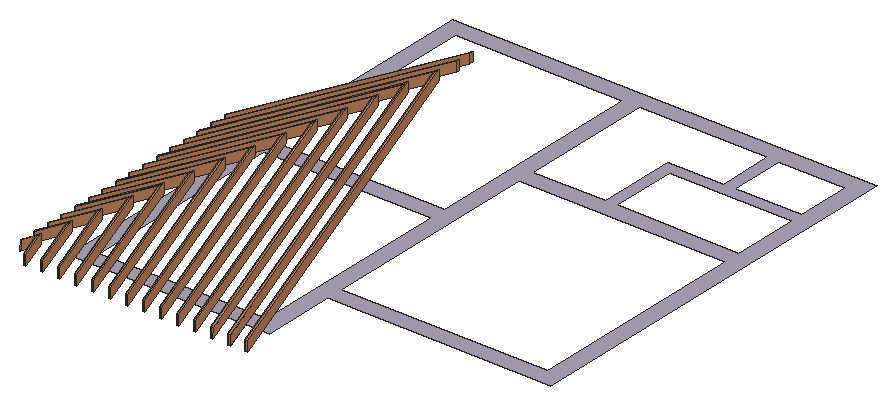
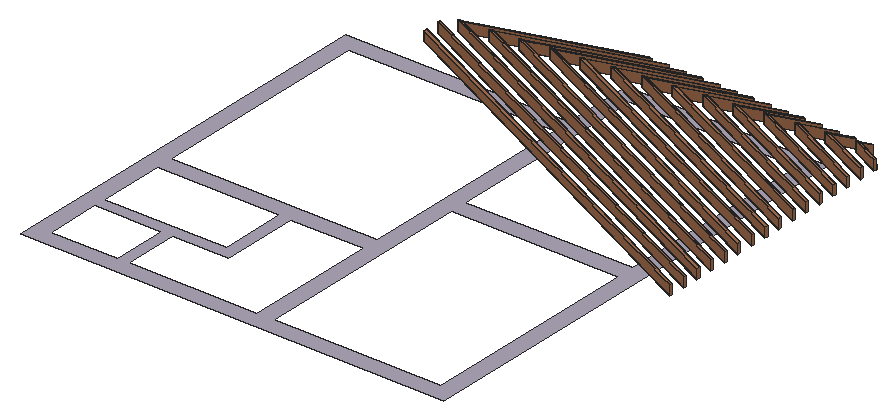
# SketchUp Ruby script. Lengths in millimetres.
U = 1.mm
M = Sketchup.active_model
def pt(a) = Geom::Point3d.new(a.map { |v| v * U })
def face(e, loops, mat)
  f = e.add_face(loops[0].map { |a| pt(a) })
  loops[1..].each { |l| e.add_face(l.map { |a| pt(a) }).erase! }
  f.material = f.back_material = mat if mat
  f
end
# faces: each face lists its corners as indices into pts; further lists are holes
def faces(e, pts, list, mat = nil) = list.each { |f| face(e, (f[0].is_a?(Array) ? f : [f]).map { |l| l.map { |i| pts[i] } }, mat) }
# xy, xz, yz: faces in a plane at the given z, y or x. An outline is a flat list of corners, or four numbers for a rectangle; further outlines are holes
def ring(l) = l.size == 4 ? [[l[0], l[1]], [l[2], l[1]], [l[2], l[3]], [l[0], l[3]]] : l.each_slice(2).to_a
def flat(e, list, mat, &to3) = list.each { |f| face(e, (f[0].is_a?(Array) ? f : [f]).map { |l| ring(l).map { |u, v| to3.(u, v) } }, mat) }
def xy(e, z, list, mat = nil) = flat(e, list, mat) { |x, y| [x, y, z] }
def xz(e, y, list, mat = nil) = flat(e, list, mat) { |x, z| [x, y, z] }
def yz(e, x, list, mat = nil) = flat(e, list, mat) { |y, z| [x, y, z] }
def lines(e, pts, list) = list.each { |a, b| e.add_line(pt(pts[a]), pt(pts[b])) }
# prism: a flat outline (further loops are holes) pulled along v
def prism(e, loops, v, mat = nil)
  f = face(e, loops, mat); d = Geom::Vector3d.new(v.map { |x| x * U })
  f.pushpull(f.normal.samedirection?(d) ? d.length : -d.length)
end
def box(e, o, s, mat = nil) = prism(e, [[o, [o[0] + s[0], o[1], o[2]], [o[0] + s[0], o[1] + s[1], o[2]], [o[0], o[1] + s[1], o[2]]]], [0, 0, s[2]], mat)
def at(x, y, z, deg = 0) = Geom::Transformation.translation(pt([x, y, z])) * Geom::Transformation.rotation(ORIGIN, Z_AXIS, deg.degrees)
def axes(o, x, y, z) = Geom::Transformation.new([*x, 0, *y, 0, *z, 0, *pt(o).to_a, 1])
def part(name) = M.definitions.add(name)
# library, detail: a bought-in or finely detailed component or shape, given as its bounding box
def library(name, o, s) = part(name).tap { |d| box(d.entities, o, s) }
def detail(e, o, s) = box(e.add_group.entities, o, s)
def put(e, d, t, mat = nil) = e.add_instance(d, t).tap { |i| i.material = mat if mat }
def group(e, t, mat = nil) = e.add_group.tap { |g| g.transformation = t; g.material = mat if mat }.entities
root = M.entities
M.materials.add("0268 AP 7144 ITALIAN IRIS").color = [172, 166, 184]
M.materials.add("[Wood Veneer 02]").color = [190, 128, 91]
c1 = part("Group163\#1")
xy(c1.entities,0,[[-381.6,-330.5,-322.7,-279.5,0,-279.5,0,-330.5]])
xy(c1.entities,152,[[-469.4,-330.5,-87.8,-330.5,-87.8,-279.5,-410.5,-279.5]])
xz(c1.entities,-330.5,[[-381.6,0,0,0,-87.8,152,-469.4,152]])
xz(c1.entities,-279.5,[[-322.7,0,-410.5,152,-87.8,152,0,0]])
p = [[-322.7,-279.5,0],[-381.6,-330.5,0],[-469.4,-330.5,152],[-410.5,-279.5,152],[0,-330.5,0],[0,-279.5,0],
  [-87.8,-279.5,152],[-87.8,-330.5,152]]
faces(c1.entities,p,[[0,1,2,3],[4,5,6,7]])
c2 = part("Group214\#1")
xy(c2.entities,0,[[-322.7,-8540.5,-381.6,-8489.5,0,-8489.5,0,-8540.5]])
xy(c2.entities,152,[[-410.5,-8540.5,-87.8,-8540.5,-87.8,-8489.5,-469.4,-8489.5]])
xz(c2.entities,-8540.5,[[-322.7,0,0,0,-87.8,152,-410.5,152]])
xz(c2.entities,-8489.5,[[-381.6,0,-469.4,152,-87.8,152,0,0]])
p = [[-322.7,-8540.5,0],[-410.5,-8540.5,152],[-469.4,-8489.5,152],[-381.6,-8489.5,0],[-87.8,-8540.5,152],[0,-8540.5,0],
  [0,-8489.5,0],[-87.8,-8489.5,152]]
faces(c2.entities,p,[[0,1,2,3],[4,5,6,7]])
c3 = part("Group165\#1")
xy(c3.entities,0,[[-733.8,-635.5,-674.9,-584.5,0,-584.5,0,-635.5]])
xy(c3.entities,152,[[-821.6,-635.5,-87.8,-635.5,-87.8,-584.5,-762.7,-584.5]])
xz(c3.entities,-635.5,[[-733.8,0,0,0,-87.8,152,-821.6,152]])
xz(c3.entities,-584.5,[[-674.9,0,-762.7,152,-87.8,152,0,0]])
p = [[-821.6,-635.5,152],[-762.7,-584.5,152],[-674.9,-584.5,0],[-733.8,-635.5,0],[-87.8,-584.5,152],[-87.8,-635.5,152],
  [0,-635.5,0],[0,-584.5,0]]
faces(c3.entities,p,[[0,1,2,3],[4,5,6,7]])
c4 = part("Group167\#1")
xy(c4.entities,0,[[-1086,-940.5,-1027.1,-889.5,0,-889.5,0,-940.5]])
xy(c4.entities,152,[[-1173.8,-940.5,-87.8,-940.5,-87.8,-889.5,-1114.9,-889.5]])
xz(c4.entities,-940.5,[[-1086,0,0,0,-87.8,152,-1173.8,152]])
xz(c4.entities,-889.5,[[-1027.1,0,-1114.9,152,-87.8,152,0,0]])
p = [[-1114.9,-889.5,152],[-1027.1,-889.5,0],[-1086,-940.5,0],[-1173.8,-940.5,152],[0,-889.5,0],[-87.8,-889.5,152],
  [-87.8,-940.5,152],[0,-940.5,0]]
faces(c4.entities,p,[[0,1,2,3],[4,5,6,7]])
c5 = part("Group216\#1")
xy(c5.entities,0,[[-674.9,-8235.5,-733.8,-8184.5,0,-8184.5,0,-8235.5]])
xy(c5.entities,152,[[-762.7,-8235.5,-87.8,-8235.5,-87.8,-8184.5,-821.6,-8184.5]])
xz(c5.entities,-8235.5,[[-674.9,0,0,0,-87.8,152,-762.7,152]])
xz(c5.entities,-8184.5,[[-733.8,0,-821.6,152,-87.8,152,0,0]])
p = [[-821.6,-8184.5,152],[-733.8,-8184.5,0],[-674.9,-8235.5,0],[-762.7,-8235.5,152],[0,-8184.5,0],[-87.8,-8184.5,152],
  [-87.8,-8235.5,152],[0,-8235.5,0]]
faces(c5.entities,p,[[0,1,2,3],[4,5,6,7]])
c6 = part("Group169\#1")
xy(c6.entities,0,[[-1438.2,-1245.5,-1379.3,-1194.5,0,-1194.5,0,-1245.5]])
xy(c6.entities,152,[[-1525.9,-1245.5,-87.8,-1245.5,-87.8,-1194.5,-1467,-1194.5]])
xz(c6.entities,-1245.5,[[-1438.2,0,0,0,-87.8,152,-1525.9,152]])
xz(c6.entities,-1194.5,[[-1379.3,0,-1467,152,-87.8,152,0,0]])
p = [[-1379.3,-1194.5,0],[-1438.2,-1245.5,0],[-1525.9,-1245.5,152],[-1467,-1194.5,152],[0,-1245.5,0],[0,-1194.5,0],
  [-87.8,-1194.5,152],[-87.8,-1245.5,152]]
faces(c6.entities,p,[[0,1,2,3],[4,5,6,7]])
c7 = part("Group171\#1")
xy(c7.entities,0,[[-1790.4,-1550.5,-1731.5,-1499.5,0,-1499.5,0,-1550.5]])
xy(c7.entities,152,[[-1878.1,-1550.5,-87.8,-1550.5,-87.8,-1499.5,-1819.2,-1499.5]])
xz(c7.entities,-1550.5,[[-1790.4,0,0,0,-87.8,152,-1878.1,152]])
xz(c7.entities,-1499.5,[[-1731.5,0,-1819.2,152,-87.8,152,0,0]])
p = [[-1819.2,-1499.5,152],[-1731.5,-1499.5,0],[-1790.4,-1550.5,0],[-1878.1,-1550.5,152],[0,-1499.5,0],[-87.8,-1499.5,152],
  [-87.8,-1550.5,152],[0,-1550.5,0]]
faces(c7.entities,p,[[0,1,2,3],[4,5,6,7]])
c8 = part("Group218\#1")
xy(c8.entities,0,[[-1027.1,-7930.5,-1086,-7879.5,0,-7879.5,0,-7930.5]])
xy(c8.entities,152,[[-1114.9,-7930.5,-87.8,-7930.5,-87.8,-7879.5,-1173.8,-7879.5]])
xz(c8.entities,-7930.5,[[-1027.1,0,0,0,-87.8,152,-1114.9,152]])
xz(c8.entities,-7879.5,[[-1086,0,-1173.8,152,-87.8,152,0,0]])
p = [[-1173.8,-7879.5,152],[-1086,-7879.5,0],[-1027.1,-7930.5,0],[-1114.9,-7930.5,152],[0,-7879.5,0],[-87.8,-7879.5,152],
  [-87.8,-7930.5,152],[0,-7930.5,0]]
faces(c8.entities,p,[[0,1,2,3],[4,5,6,7]])
c9 = part("Group173\#1")
xy(c9.entities,0,[[-2142.5,-1855.5,-2083.7,-1804.5,0,-1804.5,0,-1855.5]])
xy(c9.entities,152,[[-2230.3,-1855.5,-87.8,-1855.5,-87.8,-1804.5,-2171.4,-1804.5]])
xz(c9.entities,-1855.5,[[-2142.5,0,0,0,-87.8,152,-2230.3,152]])
xz(c9.entities,-1804.5,[[-2083.7,0,-2171.4,152,-87.8,152,0,0]])
p = [[-2083.7,-1804.5,0],[-2142.5,-1855.5,0],[-2230.3,-1855.5,152],[-2171.4,-1804.5,152],[0,-1855.5,0],[0,-1804.5,0],
  [-87.8,-1804.5,152],[-87.8,-1855.5,152]]
faces(c9.entities,p,[[0,1,2,3],[4,5,6,7]])
c10 = part("Group175\#1")
xy(c10.entities,0,[[-2494.7,-2160.5,-2435.8,-2109.5,0,-2109.5,0,-2160.5]])
xy(c10.entities,152,[[-2582.5,-2160.5,-87.8,-2160.5,-87.8,-2109.5,-2523.6,-2109.5]])
xz(c10.entities,-2160.5,[[-2494.7,0,0,0,-87.8,152,-2582.5,152]])
xz(c10.entities,-2109.5,[[-2435.8,0,-2523.6,152,-87.8,152,0,0]])
p = [[-2494.7,-2160.5,0],[-2582.5,-2160.5,152],[-2523.6,-2109.5,152],[-2435.8,-2109.5,0],[-87.8,-2160.5,152],[0,-2160.5,0],
  [0,-2109.5,0],[-87.8,-2109.5,152]]
faces(c10.entities,p,[[0,1,2,3],[4,5,6,7]])
c11 = part("Group220\#1")
xy(c11.entities,0,[[-1379.3,-7625.5,-1438.2,-7574.5,0,-7574.5,0,-7625.5]])
xy(c11.entities,152,[[-1467,-7625.5,-87.8,-7625.5,-87.8,-7574.5,-1525.9,-7574.5]])
xz(c11.entities,-7625.5,[[-1379.3,0,0,0,-87.8,152,-1467,152]])
xz(c11.entities,-7574.5,[[-1438.2,0,-1525.9,152,-87.8,152,0,0]])
p = [[-1379.3,-7625.5,0],[-1467,-7625.5,152],[-1525.9,-7574.5,152],[-1438.2,-7574.5,0],[-87.8,-7625.5,152],[0,-7625.5,0],
  [0,-7574.5,0],[-87.8,-7574.5,152]]
faces(c11.entities,p,[[0,1,2,3],[4,5,6,7]])
c12 = part("Group177\#1")
xy(c12.entities,0,[[-2846.9,-2465.5,-2788,-2414.5,0,-2414.5,0,-2465.5]])
xy(c12.entities,152,[[-2934.7,-2465.5,-87.8,-2465.5,-87.8,-2414.5,-2875.8,-2414.5]])
xz(c12.entities,-2465.5,[[-2846.9,0,0,0,-87.8,152,-2934.7,152]])
xz(c12.entities,-2414.5,[[-2788,0,-2875.8,152,-87.8,152,0,0]])
p = [[-2788,-2414.5,0],[-2846.9,-2465.5,0],[-2934.7,-2465.5,152],[-2875.8,-2414.5,152],[0,-2465.5,0],[0,-2414.5,0],
  [-87.8,-2414.5,152],[-87.8,-2465.5,152]]
faces(c12.entities,p,[[0,1,2,3],[4,5,6,7]])
c13 = part("Group179\#1")
xy(c13.entities,0,[[-3199.1,-2770.5,-3140.2,-2719.5,0,-2719.5,0,-2770.5]])
xy(c13.entities,152,[[-3286.9,-2770.5,-87.8,-2770.5,-87.8,-2719.5,-3228,-2719.5]])
xz(c13.entities,-2770.5,[[-3199.1,0,0,0,-87.8,152,-3286.9,152]])
xz(c13.entities,-2719.5,[[-3140.2,0,-3228,152,-87.8,152,0,0]])
p = [[-3228,-2719.5,152],[-3140.2,-2719.5,0],[-3199.1,-2770.5,0],[-3286.9,-2770.5,152],[0,-2719.5,0],[-87.8,-2719.5,152],
  [-87.8,-2770.5,152],[0,-2770.5,0]]
faces(c13.entities,p,[[0,1,2,3],[4,5,6,7]])
c14 = part("Group222\#1")
xy(c14.entities,0,[[-1731.5,-7320.5,-1790.4,-7269.5,0,-7269.5,0,-7320.5]])
xy(c14.entities,152,[[-1819.2,-7320.5,-87.8,-7320.5,-87.8,-7269.5,-1878.1,-7269.5]])
xz(c14.entities,-7320.5,[[-1731.5,0,0,0,-87.8,152,-1819.2,152]])
xz(c14.entities,-7269.5,[[-1790.4,0,-1878.1,152,-87.8,152,0,0]])
p = [[-1819.2,-7320.5,152],[-1878.1,-7269.5,152],[-1790.4,-7269.5,0],[-1731.5,-7320.5,0],[-87.8,-7269.5,152],[-87.8,-7320.5,152],
  [0,-7320.5,0],[0,-7269.5,0]]
faces(c14.entities,p,[[0,1,2,3],[4,5,6,7]])
c15 = part("Group181\#1")
xy(c15.entities,0,[[-3551.3,-3075.5,-3492.4,-3024.5,0,-3024.5,0,-3075.5]])
xy(c15.entities,152,[[-3639,-3075.5,-87.8,-3075.5,-87.8,-3024.5,-3580.1,-3024.5]])
xz(c15.entities,-3075.5,[[-3551.3,0,0,0,-87.8,152,-3639,152]])
xz(c15.entities,-3024.5,[[-3492.4,0,-3580.1,152,-87.8,152,0,0]])
p = [[-3639,-3075.5,152],[-3580.1,-3024.5,152],[-3492.4,-3024.5,0],[-3551.3,-3075.5,0],[-87.8,-3024.5,152],[-87.8,-3075.5,152],
  [0,-3075.5,0],[0,-3024.5,0]]
faces(c15.entities,p,[[0,1,2,3],[4,5,6,7]])
c16 = part("Group183\#1")
xy(c16.entities,0,[[-3903.5,-3380.5,-3844.6,-3329.5,0,-3329.5,0,-3380.5]])
xy(c16.entities,152,[[-3991.2,-3380.5,-87.8,-3380.5,-87.8,-3329.5,-3932.3,-3329.5]])
xz(c16.entities,-3380.5,[[-3903.5,0,0,0,-87.8,152,-3991.2,152]])
xz(c16.entities,-3329.5,[[-3844.6,0,-3932.3,152,-87.8,152,0,0]])
p = [[-3991.2,-3380.5,152],[-3932.3,-3329.5,152],[-3844.6,-3329.5,0],[-3903.5,-3380.5,0],[-87.8,-3329.5,152],[-87.8,-3380.5,152],
  [0,-3380.5,0],[0,-3329.5,0]]
faces(c16.entities,p,[[0,1,2,3],[4,5,6,7]])
c17 = part("Group224\#1")
xy(c17.entities,0,[[-2083.7,-7015.5,-2142.5,-6964.5,0,-6964.5,0,-7015.5]])
xy(c17.entities,152,[[-2171.4,-7015.5,-87.8,-7015.5,-87.8,-6964.5,-2230.3,-6964.5]])
xz(c17.entities,-7015.5,[[-2083.7,0,0,0,-87.8,152,-2171.4,152]])
xz(c17.entities,-6964.5,[[-2142.5,0,-2230.3,152,-87.8,152,0,0]])
p = [[-2142.5,-6964.5,0],[-2083.7,-7015.5,0],[-2171.4,-7015.5,152],[-2230.3,-6964.5,152],[0,-7015.5,0],[0,-6964.5,0],
  [-87.8,-6964.5,152],[-87.8,-7015.5,152]]
faces(c17.entities,p,[[0,1,2,3],[4,5,6,7]])
c18 = part("Group185\#1")
xy(c18.entities,0,[[-4255.6,-3685.5,-4196.8,-3634.5,0,-3634.5,0,-3685.5]])
xy(c18.entities,152,[[-4343.4,-3685.5,-87.8,-3685.5,-87.8,-3634.5,-4284.5,-3634.5]])
xz(c18.entities,-3685.5,[[-4255.6,0,0,0,-87.8,152,-4343.4,152]])
xz(c18.entities,-3634.5,[[-4196.8,0,-4284.5,152,-87.8,152,0,0]])
p = [[-4284.5,-3634.5,152],[-4196.8,-3634.5,0],[-4255.6,-3685.5,0],[-4343.4,-3685.5,152],[0,-3634.5,0],[-87.8,-3634.5,152],
  [-87.8,-3685.5,152],[0,-3685.5,0]]
faces(c18.entities,p,[[0,1,2,3],[4,5,6,7]])
c19 = part("Group187\#1")
xy(c19.entities,0,[[-4607.8,-3990.5,-4548.9,-3939.5,0,-3939.5,0,-3990.5]])
xy(c19.entities,152,[[-4695.6,-3990.5,-87.8,-3990.5,-87.8,-3939.5,-4636.7,-3939.5]])
xz(c19.entities,-3990.5,[[-4607.8,0,0,0,-87.8,152,-4695.6,152]])
xz(c19.entities,-3939.5,[[-4548.9,0,-4636.7,152,-87.8,152,0,0]])
p = [[-4548.9,-3939.5,0],[-4607.8,-3990.5,0],[-4695.6,-3990.5,152],[-4636.7,-3939.5,152],[0,-3990.5,0],[0,-3939.5,0],
  [-87.8,-3939.5,152],[-87.8,-3990.5,152]]
faces(c19.entities,p,[[0,1,2,3],[4,5,6,7]])
c20 = part("Group226\#1")
xy(c20.entities,0,[[-2435.8,-6710.5,-2494.7,-6659.5,0,-6659.5,0,-6710.5]])
xy(c20.entities,152,[[-2523.6,-6710.5,-87.8,-6710.5,-87.8,-6659.5,-2582.5,-6659.5]])
xz(c20.entities,-6710.5,[[-2435.8,0,0,0,-87.8,152,-2523.6,152]])
xz(c20.entities,-6659.5,[[-2494.7,0,-2582.5,152,-87.8,152,0,0]])
p = [[-2582.5,-6659.5,152],[-2494.7,-6659.5,0],[-2435.8,-6710.5,0],[-2523.6,-6710.5,152],[0,-6659.5,0],[-87.8,-6659.5,152],
  [-87.8,-6710.5,152],[0,-6710.5,0]]
faces(c20.entities,p,[[0,1,2,3],[4,5,6,7]])
c21 = part("Group189\#1")
xy(c21.entities,0,[[-4960,-4295.5,-4901.1,-4244.5,0,-4244.5,0,-4295.5]])
xy(c21.entities,152,[[-5047.8,-4295.5,-87.8,-4295.5,-87.8,-4244.5,-4988.9,-4244.5]])
xz(c21.entities,-4295.5,[[-4960,0,0,0,-87.8,152,-5047.8,152]])
xz(c21.entities,-4244.5,[[-4901.1,0,-4988.9,152,-87.8,152,0,0]])
p = [[-4901.1,-4244.5,0],[-4960,-4295.5,0],[-5047.8,-4295.5,152],[-4988.9,-4244.5,152],[0,-4295.5,0],[0,-4244.5,0],
  [-87.8,-4244.5,152],[-87.8,-4295.5,152]]
faces(c21.entities,p,[[0,1,2,3],[4,5,6,7]])
c22 = part("Group191\#1")
prism(c22.entities,[[[0,-4549.5,0],[-5092.2,-4549.5,0],[-5180,-4549.5,152],[-87.8,-4549.5,152]]],[0,-51,0])
c23 = part("Group193\#1")
prism(c23.entities,[[[-87.8,-4905.5,152],[-5180,-4905.5,152],[-5092.2,-4905.5,0],[0,-4905.5,0]]],[0,51,0])
c24 = part("Group228\#1")
xy(c24.entities,0,[[-2788,-6405.5,-2846.9,-6354.5,0,-6354.5,0,-6405.5]])
xy(c24.entities,152,[[-2875.8,-6405.5,-87.8,-6405.5,-87.8,-6354.5,-2934.7,-6354.5]])
xz(c24.entities,-6405.5,[[-2788,0,0,0,-87.8,152,-2875.8,152]])
xz(c24.entities,-6354.5,[[-2846.9,0,-2934.7,152,-87.8,152,0,0]])
p = [[-2846.9,-6354.5,0],[-2788,-6405.5,0],[-2875.8,-6405.5,152],[-2934.7,-6354.5,152],[0,-6405.5,0],[0,-6354.5,0],
  [-87.8,-6354.5,152],[-87.8,-6405.5,152]]
faces(c24.entities,p,[[0,1,2,3],[4,5,6,7]])
c25 = part("Group230\#1")
xy(c25.entities,0,[[-3140.2,-6100.5,-3199.1,-6049.5,0,-6049.5,0,-6100.5]])
xy(c25.entities,152,[[-3228,-6100.5,-87.8,-6100.5,-87.8,-6049.5,-3286.9,-6049.5]])
xz(c25.entities,-6100.5,[[-3140.2,0,0,0,-87.8,152,-3228,152]])
xz(c25.entities,-6049.5,[[-3199.1,0,-3286.9,152,-87.8,152,0,0]])
p = [[-3199.1,-6049.5,0],[-3140.2,-6100.5,0],[-3228,-6100.5,152],[-3286.9,-6049.5,152],[0,-6100.5,0],[0,-6049.5,0],
  [-87.8,-6049.5,152],[-87.8,-6100.5,152]]
faces(c25.entities,p,[[0,1,2,3],[4,5,6,7]])
c26 = part("Group232\#1")
xy(c26.entities,0,[[-3492.4,-5795.5,-3551.3,-5744.5,0,-5744.5,0,-5795.5]])
xy(c26.entities,152,[[-3580.1,-5795.5,-87.8,-5795.5,-87.8,-5744.5,-3639,-5744.5]])
xz(c26.entities,-5795.5,[[-3492.4,0,0,0,-87.8,152,-3580.1,152]])
xz(c26.entities,-5744.5,[[-3551.3,0,-3639,152,-87.8,152,0,0]])
p = [[-3492.4,-5795.5,0],[-3580.1,-5795.5,152],[-3639,-5744.5,152],[-3551.3,-5744.5,0],[-87.8,-5795.5,152],[0,-5795.5,0],
  [0,-5744.5,0],[-87.8,-5744.5,152]]
faces(c26.entities,p,[[0,1,2,3],[4,5,6,7]])
c27 = part("Group234\#1")
xy(c27.entities,0,[[-3844.6,-5490.5,-3903.5,-5439.5,0,-5439.5,0,-5490.5]])
xy(c27.entities,152,[[-3932.3,-5490.5,-87.8,-5490.5,-87.8,-5439.5,-3991.2,-5439.5]])
xz(c27.entities,-5490.5,[[-3844.6,0,0,0,-87.8,152,-3932.3,152]])
xz(c27.entities,-5439.5,[[-3903.5,0,-3991.2,152,-87.8,152,0,0]])
p = [[-3991.2,-5439.5,152],[-3903.5,-5439.5,0],[-3844.6,-5490.5,0],[-3932.3,-5490.5,152],[0,-5439.5,0],[-87.8,-5439.5,152],
  [-87.8,-5490.5,152],[0,-5490.5,0]]
faces(c27.entities,p,[[0,1,2,3],[4,5,6,7]])
c28 = part("Group236\#1")
xy(c28.entities,0,[[-4196.8,-5185.5,-4255.6,-5134.5,0,-5134.5,0,-5185.5]])
xy(c28.entities,152,[[-4284.5,-5185.5,-87.8,-5185.5,-87.8,-5134.5,-4343.4,-5134.5]])
xz(c28.entities,-5185.5,[[-4196.8,0,0,0,-87.8,152,-4284.5,152]])
xz(c28.entities,-5134.5,[[-4255.6,0,-4343.4,152,-87.8,152,0,0]])
p = [[-4255.6,-5134.5,0],[-4196.8,-5185.5,0],[-4284.5,-5185.5,152],[-4343.4,-5134.5,152],[0,-5185.5,0],[0,-5134.5,0],
  [-87.8,-5134.5,152],[-87.8,-5185.5,152]]
faces(c28.entities,p,[[0,1,2,3],[4,5,6,7]])
c29 = part("Group238\#1")
xy(c29.entities,0,[[-4548.9,-4880.5,-4607.8,-4829.5,0,-4829.5,0,-4880.5]])
xy(c29.entities,152,[[-4636.7,-4880.5,-87.8,-4880.5,-87.8,-4829.5,-4695.6,-4829.5]])
xz(c29.entities,-4880.5,[[-4548.9,0,0,0,-87.8,152,-4636.7,152]])
xz(c29.entities,-4829.5,[[-4607.8,0,-4695.6,152,-87.8,152,0,0]])
p = [[-4636.7,-4880.5,152],[-4695.6,-4829.5,152],[-4607.8,-4829.5,0],[-4548.9,-4880.5,0],[-87.8,-4829.5,152],[-87.8,-4880.5,152],
  [0,-4880.5,0],[0,-4829.5,0]]
faces(c29.entities,p,[[0,1,2,3],[4,5,6,7]])
c30 = part("Group240\#1")
xy(c30.entities,0,[[-4901.1,-4575.5,-4960,-4524.5,0,-4524.5,0,-4575.5]])
xy(c30.entities,152,[[-4988.9,-4575.5,-87.8,-4575.5,-87.8,-4524.5,-5047.8,-4524.5]])
xz(c30.entities,-4575.5,[[-4901.1,0,0,0,-87.8,152,-4988.9,152]])
xz(c30.entities,-4524.5,[[-4960,0,-5047.8,152,-87.8,152,0,0]])
p = [[-5047.8,-4524.5,152],[-4960,-4524.5,0],[-4901.1,-4575.5,0],[-4988.9,-4575.5,152],[0,-4524.5,0],[-87.8,-4524.5,152],
  [-87.8,-4575.5,152],[0,-4575.5,0]]
faces(c30.entities,p,[[0,1,2,3],[4,5,6,7]])
xy(root,3149.6,[[[1913.3,1897,5513.3,1897,5513.3,3197,9513.3,3197,9513.3,10497,1913.3,10497],[5513.3,3497,5513.3,10197,7813.3,10197,7813.3,9197,6813.3,9197,6813.3,7797,5513.3,7797,5513.3,7497,9213.3,7497,9213.3,3497],[2213.3,6197,5213.3,10197],[2213.3,2197,5213.3,5897],[7013.3,7797,9213.3,8997],[8013.3,9197,9213.3,10197]]],"0268 AP 7144 ITALIAN IRIS")
put(root,c1,axes([1303.3,1287,3149.6],[-0.86603,0,-0.5],[0,-1,0],[-0.5,0,0.86603]),"[Wood Veneer 02]")
put(root,c2,axes([10123.3,1287,3149.6],[0,-0.86603,-0.5],[1,0,0],[0,-0.5,0.86603]),"[Wood Veneer 02]")
put(root,c3,axes([1303.3,1287,3149.6],[-0.86603,0,-0.5],[0,-1,0],[-0.5,0,0.86603]),"[Wood Veneer 02]")
put(root,c4,axes([1303.3,1287,3149.6],[-0.86603,0,-0.5],[0,-1,0],[-0.5,0,0.86603]),"[Wood Veneer 02]")
put(root,c5,axes([10123.3,1287,3149.6],[0,-0.86603,-0.5],[1,0,0],[0,-0.5,0.86603]),"[Wood Veneer 02]")
put(root,c6,axes([1303.3,1287,3149.6],[-0.86603,0,-0.5],[0,-1,0],[-0.5,0,0.86603]),"[Wood Veneer 02]")
put(root,c7,axes([1303.3,1287,3149.6],[-0.86603,0,-0.5],[0,-1,0],[-0.5,0,0.86603]),"[Wood Veneer 02]")
put(root,c8,axes([10123.3,1287,3149.6],[0,-0.86603,-0.5],[1,0,0],[0,-0.5,0.86603]),"[Wood Veneer 02]")
put(root,c9,axes([1303.3,1287,3149.6],[-0.86603,0,-0.5],[0,-1,0],[-0.5,0,0.86603]),"[Wood Veneer 02]")
put(root,c10,axes([1303.3,1287,3149.6],[-0.86603,0,-0.5],[0,-1,0],[-0.5,0,0.86603]),"[Wood Veneer 02]")
put(root,c11,axes([10123.3,1287,3149.6],[0,-0.86603,-0.5],[1,0,0],[0,-0.5,0.86603]),"[Wood Veneer 02]")
put(root,c12,axes([1303.3,1287,3149.6],[-0.86603,0,-0.5],[0,-1,0],[-0.5,0,0.86603]),"[Wood Veneer 02]")
put(root,c13,axes([1303.3,1287,3149.6],[-0.86603,0,-0.5],[0,-1,0],[-0.5,0,0.86603]),"[Wood Veneer 02]")
put(root,c14,axes([10123.3,1287,3149.6],[0,-0.86603,-0.5],[1,0,0],[0,-0.5,0.86603]),"[Wood Veneer 02]")
put(root,c15,axes([1303.3,1287,3149.6],[-0.86603,0,-0.5],[0,-1,0],[-0.5,0,0.86603]),"[Wood Veneer 02]")
put(root,c16,axes([1303.3,1287,3149.6],[-0.86603,0,-0.5],[0,-1,0],[-0.5,0,0.86603]),"[Wood Veneer 02]")
put(root,c17,axes([10123.3,1287,3149.6],[0,-0.86603,-0.5],[1,0,0],[0,-0.5,0.86603]),"[Wood Veneer 02]")
put(root,c18,axes([1303.3,1287,3149.6],[-0.86603,0,-0.5],[0,-1,0],[-0.5,0,0.86603]),"[Wood Veneer 02]")
put(root,c19,axes([1303.3,1287,3149.6],[-0.86603,0,-0.5],[0,-1,0],[-0.5,0,0.86603]),"[Wood Veneer 02]")
put(root,c20,axes([10123.3,1287,3149.6],[0,-0.86603,-0.5],[1,0,0],[0,-0.5,0.86603]),"[Wood Veneer 02]")
put(root,c21,axes([1303.3,1287,3149.6],[-0.86603,0,-0.5],[0,-1,0],[-0.5,0,0.86603]),"[Wood Veneer 02]")
put(root,c22,axes([1303.3,1287,3149.6],[-0.86603,0,-0.5],[0,-1,0],[-0.5,0,0.86603]),"[Wood Veneer 02]")
put(root,c23,axes([1303.3,1287,3149.6],[-0.86603,0,-0.5],[0,-1,0],[-0.5,0,0.86603]),"[Wood Veneer 02]")
put(root,c24,axes([10123.3,1287,3149.6],[0,-0.86603,-0.5],[1,0,0],[0,-0.5,0.86603]),"[Wood Veneer 02]")
put(root,c25,axes([10123.3,1287,3149.6],[0,-0.86603,-0.5],[1,0,0],[0,-0.5,0.86603]),"[Wood Veneer 02]")
put(root,c26,axes([10123.3,1287,3149.6],[0,-0.86603,-0.5],[1,0,0],[0,-0.5,0.86603]),"[Wood Veneer 02]")
put(root,c27,axes([10123.3,1287,3149.6],[0,-0.86603,-0.5],[1,0,0],[0,-0.5,0.86603]),"[Wood Veneer 02]")
put(root,c28,axes([10123.3,1287,3149.6],[0,-0.86603,-0.5],[1,0,0],[0,-0.5,0.86603]),"[Wood Veneer 02]")
put(root,c29,axes([10123.3,1287,3149.6],[0,-0.86603,-0.5],[1,0,0],[0,-0.5,0.86603]),"[Wood Veneer 02]")
put(root,c30,axes([10123.3,1287,3149.6],[0,-0.86603,-0.5],[1,0,0],[0,-0.5,0.86603]),"[Wood Veneer 02]")
